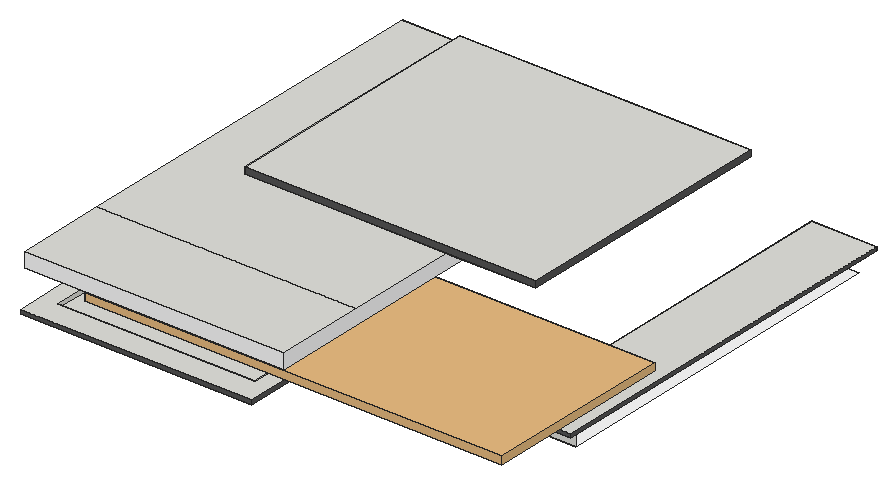
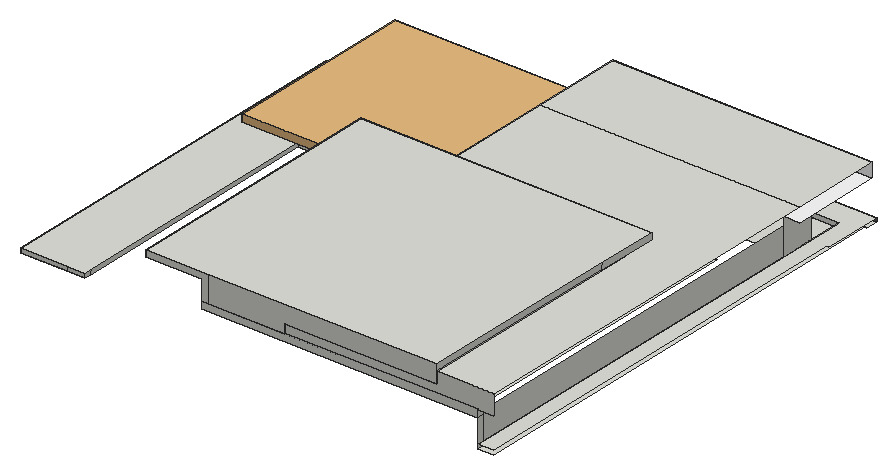
# SketchUp Ruby script. Lengths in inches.
U = 1.inch
M = Sketchup.active_model
def pt(a) = Geom::Point3d.new(a.map { |v| v * U })
def face(e, loops, mat)
  f = e.add_face(loops[0].map { |a| pt(a) })
  loops[1..].each { |l| e.add_face(l.map { |a| pt(a) }).erase! }
  f.material = f.back_material = mat if mat
  f
end
# faces: each face lists its corners as indices into pts; further lists are holes
def faces(e, pts, list, mat = nil) = list.each { |f| face(e, (f[0].is_a?(Array) ? f : [f]).map { |l| l.map { |i| pts[i] } }, mat) }
# xy, xz, yz: faces in a plane at the given z, y or x. An outline is a flat list of corners, or four numbers for a rectangle; further outlines are holes
def ring(l) = l.size == 4 ? [[l[0], l[1]], [l[2], l[1]], [l[2], l[3]], [l[0], l[3]]] : l.each_slice(2).to_a
def flat(e, list, mat, &to3) = list.each { |f| face(e, (f[0].is_a?(Array) ? f : [f]).map { |l| ring(l).map { |u, v| to3.(u, v) } }, mat) }
def xy(e, z, list, mat = nil) = flat(e, list, mat) { |x, y| [x, y, z] }
def xz(e, y, list, mat = nil) = flat(e, list, mat) { |x, z| [x, y, z] }
def yz(e, x, list, mat = nil) = flat(e, list, mat) { |y, z| [x, y, z] }
def lines(e, pts, list) = list.each { |a, b| e.add_line(pt(pts[a]), pt(pts[b])) }
# prism: a flat outline (further loops are holes) pulled along v
def prism(e, loops, v, mat = nil)
  f = face(e, loops, mat); d = Geom::Vector3d.new(v.map { |x| x * U })
  f.pushpull(f.normal.samedirection?(d) ? d.length : -d.length)
end
def box(e, o, s, mat = nil) = prism(e, [[o, [o[0] + s[0], o[1], o[2]], [o[0] + s[0], o[1] + s[1], o[2]], [o[0], o[1] + s[1], o[2]]]], [0, 0, s[2]], mat)
def at(x, y, z, deg = 0) = Geom::Transformation.translation(pt([x, y, z])) * Geom::Transformation.rotation(ORIGIN, Z_AXIS, deg.degrees)
def axes(o, x, y, z) = Geom::Transformation.new([*x, 0, *y, 0, *z, 0, *pt(o).to_a, 1])
def part(name) = M.definitions.add(name)
# library, detail: a bought-in or finely detailed component or shape, given as its bounding box
def library(name, o, s) = part(name).tap { |d| box(d.entities, o, s) }
def detail(e, o, s) = box(e.add_group.entities, o, s)
def put(e, d, t, mat = nil) = e.add_instance(d, t).tap { |i| i.material = mat if mat }
def group(e, t, mat = nil) = e.add_group.tap { |g| g.transformation = t; g.material = mat if mat }.entities
root = M.entities
M.materials.add("[Color M00]").color = [255, 255, 255]
M.materials.add("[Color M06]").color = [86, 86, 86]
c1 = library("Mesh Light\#4",[-0.5,-0.5,-0.1],[1,1,0.2])
c2 = part("Group\#24")
xy(c2.entities,0,[[203.13,95.41,201.58,95.62,200.13,96.22,198.89,97.17,197.9375,98.41,197.34,99.86,197.13,101.41,197.34,102.96,197.9375,104.41,198.89,105.65,200.13,106.61,201.58,107.21,203.13,107.41,204.6875,107.21,206.13,106.61,207.375,105.65,208.33,104.41,208.93,102.96,209.13,101.41,208.93,99.86,208.33,98.41,207.375,97.17,206.13,96.22,204.6875,95.62],[281.57,95.41,280.02,95.62,278.57,96.22,277.33,97.17,276.375,98.41,275.77,99.86,275.57,101.41,275.77,102.96,276.375,104.41,277.33,105.65,278.57,106.61,280.02,107.21,281.57,107.41,283.125,107.21,284.57,106.61,285.8125,105.65,286.77,104.41,287.37,102.96,287.57,101.41,287.37,99.86,286.77,98.41,285.8125,97.17,284.57,96.22,283.125,95.62],[350.95,95.41,349.39,95.62,347.95,96.22,346.7,97.17,345.75,98.41,345.15,99.86,344.95,101.41,345.15,102.96,345.75,104.41,346.7,105.65,347.95,106.61,349.39,107.21,350.95,107.41,352.5,107.21,353.95,106.61,355.1875,105.65,356.14,104.41,356.74,102.96,356.95,101.41,356.74,99.86,356.14,98.41,355.1875,97.17,353.95,96.22,352.5,95.62],[376,162.85,374.44,163.05,373,163.65,371.75,164.6,370.8,165.85,370.2,167.29,370,168.85,370.2,170.4,370.8,171.85,371.75,173.09,373,174.04,374.44,174.64,376,174.85,377.55,174.64,379,174.04,380.24,173.09,381.19,171.85,381.79,170.4,382,168.85,381.79,167.29,381.19,165.85,380.24,164.6,379,163.65,377.55,163.05]],"[Color M00]")
xy(c2.entities,33.4375,[[6,0,4.45,0.2,3,0.8,1.76,1.76,0.8,3,0.2,4.45,0,6,0.2,7.55,0.8,9,1.76,10.24,3,11.2,4.45,11.8,6,12,7.55,11.8,9,11.2,10.24,10.24,11.2,9,11.8,7.55,12,6,11.8,4.45,11.2,3,10.24,1.76,9,0.8,7.55,0.2],[83.125,0,81.57,0.2,80.125,0.8,78.88,1.76,77.93,3,77.33,4.45,77.125,6,77.33,7.55,77.93,9,78.88,10.24,80.125,11.2,81.57,11.8,83.125,12,84.68,11.8,86.125,11.2,87.37,10.24,88.32,9,88.92,7.55,89.125,6,88.92,4.45,88.32,3,87.37,1.76,86.125,0.8,84.68,0.2],[166.6875,0,165.13,0.2,163.6875,0.8,162.44,1.76,161.49,3,160.89,4.45,160.6875,6,160.89,7.55,161.49,9,162.44,10.24,163.6875,11.2,165.13,11.8,166.6875,12,168.24,11.8,169.6875,11.2,170.93,10.24,171.88,9,172.48,7.55,172.6875,6,172.48,4.45,171.88,3,170.93,1.76,169.6875,0.8,168.24,0.2],[166.6875,88.9375,165.13,89.14,163.6875,89.74,162.44,90.69,161.49,91.9375,160.89,93.38,160.6875,94.9375,160.89,96.49,161.49,97.9375,162.44,99.18,163.6875,100.13,165.13,100.73,166.6875,100.9375,168.24,100.73,169.6875,100.13,170.93,99.18,171.88,97.9375,172.48,96.49,172.6875,94.9375,172.48,93.38,171.88,91.9375,170.93,90.69,169.6875,89.74,168.24,89.14]],"[Color M00]")
put(c2.entities,c1,axes([191,87.42,16.72],[382.99758,0,0],[0,175.84579,0],[0,0,34.4375]))
c3 = library("Group\#23",[-0.5,-0.5,-0.1],[13,110.375,0.2])
xy(root,270.375,[[2956.13,1581.1,3168.57,1592.1],[2957.51,1592.1,2957.51,2018.36,2972.24,2018.36,2972.24,1604.38,3153.06,1604.38,3153.06,1703.22,3162.07,1703.22,3162.07,1592.1],[3162.07,1592.1,3168.57,1636.04],[2972.24,1604.38,3153.06,1604.38,3153.06,1703.22,3149.44,1703.22,3149.44,1659.57,2972.24,1659.57],[3162.07,1636.04,3168.57,1728.29],
  [3149.44,1703.22,3162.07,1773.67]])
xy(root,274.0625,[[2956.13,1581.1,3168.57,1581.1,3168.57,1673.72,3162.07,1673.72,3162.07,1703.22,3153.06,1703.22,3153.06,1604.38,2972.24,1604.38,2972.24,2018.36,2957.51,2018.36,2957.51,1636.04,2956.13,1636.04],[3162.07,1673.72,3168.57,1728.29]])
xy(root,274.0625,[[[3168.57,1673.72,3168.57,1728.29,3352.26,1728.29,3352.26,1998.71,3392.88,1998.71,3392.88,1673.72],[3203.78,1695.77,3205.34,1695.97,3206.78,1696.57,3208.03,1697.52,3208.98,1698.77,3209.58,1700.21,3209.78,1701.77,3209.58,1703.32,3208.98,1704.77,3208.03,1706.01,3206.78,1706.96,3205.34,1707.5625,3203.78,1707.77,3202.23,1707.5625,3200.78,1706.96,3199.54,1706.01,3198.59,1704.77,3197.99,1703.32,3197.78,1701.77,3197.99,1700.21,3198.59,1698.77,3199.54,1697.52,3200.78,1696.57,3202.23,1695.97],[3282.22,1695.77,3283.77,1695.97,3285.22,1696.57,3286.46,1697.52,3287.42,1698.77,3288.02,1700.21,3288.22,1701.77,3288.02,1703.32,3287.42,1704.77,3286.46,1706.01,3285.22,1706.96,3283.77,1707.5625,3282.22,1707.77,3280.67,1707.5625,3279.22,1706.96,3277.98,1706.01,3277.03,1704.77,3276.43,1703.32,3276.22,1701.77,3276.43,1700.21,3277.03,1698.77,3277.98,1697.52,3279.22,1696.57,3280.67,1695.97],[3351.6,1695.77,3353.15,1695.97,3354.6,1696.57,3355.84,1697.52,3356.79,1698.77,3357.39,1700.21,3357.6,1701.77,3357.39,1703.32,3356.79,1704.77,3355.84,1706.01,3354.6,1706.96,3353.15,1707.5625,3351.6,1707.77,3350.04,1707.5625,3348.6,1706.96,3347.35,1706.01,3346.4,1704.77,3345.8,1703.32,3345.6,1701.77,3345.8,1700.21,3346.4,1698.77,3347.35,1697.52,3348.6,1696.57,3350.04,1695.97],[3376.65,1843.64,3378.2,1843.84,3379.65,1844.44,3380.89,1845.39,3381.85,1846.64,3382.44,1848.08,3382.65,1849.64,3382.44,1851.19,3381.85,1852.64,3380.89,1853.88,3379.65,1854.83,3378.2,1855.43,3376.65,1855.64,3375.1,1855.43,3373.65,1854.83,3372.41,1853.88,3371.45,1852.64,3370.85,1851.19,3370.65,1849.64,3370.85,1848.08,3371.45,1846.64,3372.41,1845.39,3373.65,1844.44,3375.1,1843.84],[3376.65,1763.2,3378.2,1763.4,3379.65,1764,3380.89,1764.96,3381.85,1766.2,3382.44,1767.65,3382.65,1769.2,3382.44,1770.75,3381.85,1772.2,3380.89,1773.44,3379.65,1774.4,3378.2,1774.99,3376.65,1775.2,3375.1,1774.99,3373.65,1774.4,3372.41,1773.44,3371.45,1772.2,3370.85,1770.75,3370.65,1769.2,3370.85,1767.65,3371.45,1766.2,3372.41,1764.96,3373.65,1764,3375.1,1763.4],[3376.65,1941.01,3378.2,1941.22,3379.65,1941.82,3380.89,1942.77,3381.85,1944.01,3382.44,1945.46,3382.65,1947.01,3382.44,1948.56,3381.85,1950.01,3380.89,1951.25,3379.65,1952.21,3378.2,1952.81,3376.65,1953.01,3375.1,1952.81,3373.65,1952.21,3372.41,1951.25,3371.45,1950.01,3370.85,1948.56,3370.65,1947.01,3370.85,1945.46,3371.45,1944.01,3372.41,1942.77,3373.65,1941.82,3375.1,1941.22]]],"[Color M00]")
xy(root,283.9375,[[3162.07,1667.47,3392.88,1673.72],[3162.07,1673.72,3162.07,1773.67,3333.43,1773.67,3333.43,2018.36,3392.88,2018.36,3392.88,1673.72]])
xy(root,287.375,[[3162.07,1667.47,3392.88,1667.47,3392.88,2018.36,3333.43,2018.36,3333.43,1773.67,3162.07,1773.67]])
xy(root,295.8125,[[2982.55,1730.8,2982.55,2011.98,3149.44,2011.98,3149.44,1851.54,3139.92,1851.54,3139.92,1730.8],[3149.44,1851.54,3219.88,2011.98]])
xy(root,302.5625,[[2972.24,2011.98,3149.44,2018.36],[3149.44,2011.98,3219.88,2018.36]])
xy(root,307.5,[[[2957.51,1584.22,2957.51,1667.53,2972.24,1667.53,2972.24,1636.22,3149.44,1636.22,3149.44,1829.17,3195.88,1829.17,3195.88,1584.22],[3006.65,1600.35,3008.2,1600.56,3009.65,1601.16,3010.89,1602.11,3011.85,1603.35,3012.45,1604.8,3012.65,1606.35,3012.45,1607.91,3011.85,1609.35,3010.89,1610.6,3009.65,1611.55,3008.2,1612.15,3006.65,1612.35,3005.1,1612.15,3003.65,1611.55,3002.41,1610.6,3001.46,1609.35,3000.86,1607.91,3000.65,1606.35,3000.86,1604.8,3001.46,1603.35,3002.41,1602.11,3003.65,1601.16,3005.1,1600.56],[3083.78,1600.35,3085.33,1600.56,3086.78,1601.16,3088.02,1602.11,3088.97,1603.35,3089.57,1604.8,3089.78,1606.35,3089.57,1607.91,3088.97,1609.35,3088.02,1610.6,3086.78,1611.55,3085.33,1612.15,3083.78,1612.35,3082.22,1612.15,3080.78,1611.55,3079.53,1610.6,3078.58,1609.35,3077.98,1607.91,3077.78,1606.35,3077.98,1604.8,3078.58,1603.35,3079.53,1602.11,3080.78,1601.16,3082.22,1600.56],[3167.34,1689.29,3168.89,1689.5,3170.34,1690.09,3171.58,1691.05,3172.54,1692.29,3173.13,1693.74,3173.34,1695.29,3173.13,1696.84,3172.54,1698.29,3171.58,1699.53,3170.34,1700.49,3168.89,1701.09,3167.34,1701.29,3165.79,1701.09,3164.34,1700.49,3163.1,1699.53,3162.14,1698.29,3161.54,1696.84,3161.34,1695.29,3161.54,1693.74,3162.14,1692.29,3163.1,1691.05,3164.34,1690.09,3165.79,1689.5],[3167.34,1600.35,3168.89,1600.56,3170.34,1601.16,3171.58,1602.11,3172.54,1603.35,3173.13,1604.8,3173.34,1606.35,3173.13,1607.91,3172.54,1609.35,3171.58,1610.6,3170.34,1611.55,3168.89,1612.15,3167.34,1612.35,3165.79,1612.15,3164.34,1611.55,3163.1,1610.6,3162.14,1609.35,3161.54,1607.91,3161.34,1606.35,3161.54,1604.8,3162.14,1603.35,3163.1,1602.11,3164.34,1601.16,3165.79,1600.56]]],"[Color M00]")
xy(root,310.3125,[[3009.88,1829.17,3149.44,2018.36]])
xy(root,320.75,[[2957.51,1584.22,3195.88,1667.53],[2957.51,1667.53,3195.88,1667.53,3195.88,1771.54,3009.88,1771.54,3009.88,2018.36,2957.51,2018.36],[3195.88,1771.54,3195.88,1829.17,3225.88,1829.17,3225.88,2018.36,3277.44,2018.36,3277.44,1771.54]])
xy(root,326.5,[[3009.88,1771.54,3277.44,2018.36]])
xz(root,1581.1,[[2956.13,270.375,3168.57,274.0625]],"[Color M06]")
xz(root,1584.22,[[2957.51,307.5,3195.88,320.75]],"[Color M00]")
xz(root,1604.38,[[2972.24,270.375,3153.06,274.0625]])
xz(root,1667.47,[[3162.07,283.9375,3392.88,287.375]],"[Color M06]")
xz(root,1673.72,[[3162.07,274.0625,3392.88,283.9375]])
xz(root,1703.22,[[3153.06,270.375,3162.07,274.0625]])
xz(root,1771.54,[[3009.88,320.75,3277.44,326.5]],"[Color M06]")
xz(root,1773.67,[[3162.07,283.9375,3333.43,287.375]])
xz(root,1829.17,[[3149.44,307.5,3195.88,310.3125]])
xz(root,2011.98,[[2972.24,295.8125,3149.44,302.5625],[3149.44,295.8125,3219.88,302.5625]])
xz(root,2018.36,[[3333.43,283.9375,3349.13,287.375],[3349.13,283.9375,3392.88,287.375],[2972.24,295.8125,3225.88,302.5625],[2957.51,302.5625,2957.51,320.75,3009.88,320.75,3009.88,310.3125,3149.44,310.3125,3149.44,302.5625],[3149.44,302.5625,3149.44,310.3125,3009.88,310.3125,3009.88,326.5,3219.88,326.5,3219.88,302.5625],
  [3219.88,302.5625,3219.88,326.5,3277.44,326.5,3277.44,320.75,3225.88,320.75,3225.88,302.5625]])
yz(root,2972.24,[[1604.38,270.375,1636.22,274.0625],[1636.22,270.375,1659.57,274.0625],[1659.57,270.375,1667.53,274.0625],[1667.53,270.375,2011.98,274.0625],[2011.98,270.375,2018.36,274.0625],
  [1636.22,274.0625,1667.53,307.5],[1667.53,274.0625,2011.98,299.625],[2011.98,274.0625,2018.36,295.8125],[2011.98,295.8125,2018.36,302.5625]])
yz(root,3009.88,[[1801.17,310.3125,1829.17,320.75],[1829.17,310.3125,2018.36,320.75],[1771.54,320.75,1829.17,326.5],[1829.17,320.75,2018.36,326.5]])
yz(root,3149.44,[[1829.17,295.8125,2011.98,302.5625],[1829.17,302.5625,2018.36,310.3125]])
yz(root,3153.06,[[1604.38,270.375,1703.22,274.0625]])
yz(root,3162.07,[[1728.29,270.375,1728.29,274.0625,1673.72,274.0625,1673.72,283.9375,1773.67,283.9375,1773.67,270.375],[1703.22,270.375,1728.29,274.0625],[1667.47,283.9375,1773.67,287.375]])
yz(root,3168.57,[[1581.1,270.375,1728.29,274.0625]],"[Color M06]")
yz(root,3195.88,[[1584.22,307.5,1829.17,320.75]],"[Color M00]")
yz(root,3277.44,[[1771.54,320.75,2018.36,326.5]],"[Color M06]")
yz(root,3333.43,[[1773.67,283.9375,2011.98,287.375],[2011.98,283.9375,2018.36,287.375]])
yz(root,3392.88,[[1667.47,283.9375,2018.36,287.375]],"[Color M06]")
p = [[3203.78,1695.77,274.0625],[3202.23,1695.97,274.0625],[3202.23,1695.97,274.75],[3203.78,1695.77,274.75],[3205.34,1695.97,274.0625],[3205.34,1695.97,274.75],
  [3282.22,1695.77,274.0625],[3280.67,1695.97,274.0625],[3280.67,1695.97,274.75],[3282.22,1695.77,274.75],[3283.77,1695.97,274.0625],[3283.77,1695.97,274.75],
  [3351.6,1695.77,274.0625],[3350.04,1695.97,274.0625],[3350.04,1695.97,274.75],[3351.6,1695.77,274.75],[3353.15,1695.97,274.0625],[3353.15,1695.97,274.75],
  [3200.78,1696.57,274.0625],[3200.78,1696.57,274.75],[3206.78,1696.57,274.0625],[3206.78,1696.57,274.75],[3279.22,1696.57,274.0625],[3279.22,1696.57,274.75],
  [3285.22,1696.57,274.0625],[3285.22,1696.57,274.75],[3348.6,1696.57,274.0625],[3348.6,1696.57,274.75],[3354.6,1696.57,274.0625],[3354.6,1696.57,274.75],
  [3199.54,1697.52,274.0625],[3199.54,1697.52,274.75],[3208.03,1697.52,274.0625],[3208.03,1697.52,274.75],[3277.98,1697.52,274.0625],[3277.98,1697.52,274.75],
  [3286.46,1697.52,274.0625],[3286.46,1697.52,274.75],[3347.35,1697.52,274.0625],[3347.35,1697.52,274.75],[3355.84,1697.52,274.0625],[3355.84,1697.52,274.75],
  [3198.59,1698.77,274.0625],[3198.59,1698.77,274.75],[3208.98,1698.77,274.0625],[3208.98,1698.77,274.75],[3277.03,1698.77,274.0625],[3277.03,1698.77,274.75],
  [3287.42,1698.77,274.0625],[3287.42,1698.77,274.75],[3346.4,1698.77,274.0625],[3346.4,1698.77,274.75],[3356.79,1698.77,274.0625],[3356.79,1698.77,274.75],
  [3197.99,1700.21,274.0625],[3197.99,1700.21,274.75],[3209.58,1700.21,274.0625],[3209.58,1700.21,274.75],[3276.43,1700.21,274.0625],[3276.43,1700.21,274.75],
  [3288.02,1700.21,274.0625],[3288.02,1700.21,274.75],[3345.8,1700.21,274.0625],[3345.8,1700.21,274.75],[3357.39,1700.21,274.0625],[3357.39,1700.21,274.75],
  [3197.78,1701.77,274.0625],[3197.78,1701.77,274.75],[3209.78,1701.77,274.0625],[3209.78,1701.77,274.75],[3276.22,1701.77,274.0625],[3276.22,1701.77,274.75],
  [3288.22,1701.77,274.0625],[3288.22,1701.77,274.75],[3345.6,1701.77,274.0625],[3345.6,1701.77,274.75],[3357.6,1701.77,274.0625],[3357.6,1701.77,274.75],
  [3197.99,1703.32,274.0625],[3197.99,1703.32,274.75],[3209.58,1703.32,274.0625],[3209.58,1703.32,274.75],[3276.43,1703.32,274.0625],[3276.43,1703.32,274.75],
  [3288.02,1703.32,274.0625],[3288.02,1703.32,274.75],[3345.8,1703.32,274.0625],[3345.8,1703.32,274.75],[3357.39,1703.32,274.0625],[3357.39,1703.32,274.75],
  [3198.59,1704.77,274.0625],[3198.59,1704.77,274.75],[3208.98,1704.77,274.0625],[3208.98,1704.77,274.75],[3277.03,1704.77,274.0625],[3277.03,1704.77,274.75],
  [3287.42,1704.77,274.0625],[3287.42,1704.77,274.75],[3346.4,1704.77,274.0625],[3346.4,1704.77,274.75],[3356.79,1704.77,274.0625],[3356.79,1704.77,274.75],
  [3199.54,1706.01,274.0625],[3199.54,1706.01,274.75],[3208.03,1706.01,274.0625],[3208.03,1706.01,274.75],[3277.98,1706.01,274.0625],[3277.98,1706.01,274.75],
  [3286.46,1706.01,274.0625],[3286.46,1706.01,274.75],[3347.35,1706.01,274.0625],[3347.35,1706.01,274.75],[3355.84,1706.01,274.0625],[3355.84,1706.01,274.75],
  [3200.78,1706.96,274.0625],[3200.78,1706.96,274.75],[3206.78,1706.96,274.0625],[3206.78,1706.96,274.75],[3279.22,1706.96,274.0625],[3279.22,1706.96,274.75],
  [3285.22,1706.96,274.0625],[3285.22,1706.96,274.75],[3348.6,1706.96,274.0625],[3348.6,1706.96,274.75],[3354.6,1706.96,274.0625],[3354.6,1706.96,274.75],
  [3202.23,1707.5625,274.0625],[3202.23,1707.5625,274.75],[3205.34,1707.5625,274.0625],[3205.34,1707.5625,274.75],[3280.67,1707.5625,274.0625],[3280.67,1707.5625,274.75],
  [3283.77,1707.5625,274.0625],[3283.77,1707.5625,274.75],[3350.04,1707.5625,274.0625],[3350.04,1707.5625,274.75],[3353.15,1707.5625,274.0625],[3353.15,1707.5625,274.75],
  [3203.78,1707.77,274.0625],[3203.78,1707.77,274.75],[3282.22,1707.77,274.0625],[3282.22,1707.77,274.75],[3351.6,1707.77,274.0625],[3351.6,1707.77,274.75],
  [3376.65,1763.2,274.0625],[3375.1,1763.4,274.0625],[3375.1,1763.4,274.75],[3376.65,1763.2,274.75],[3378.2,1763.4,274.0625],[3378.2,1763.4,274.75],
  [3373.65,1764,274.0625],[3373.65,1764,274.75],[3379.65,1764,274.0625],[3379.65,1764,274.75],[3372.41,1764.96,274.0625],[3372.41,1764.96,274.75],
  [3380.89,1764.96,274.0625],[3380.89,1764.96,274.75],[3371.45,1766.2,274.0625],[3371.45,1766.2,274.75],[3381.85,1766.2,274.0625],[3381.85,1766.2,274.75],
  [3370.85,1767.65,274.0625],[3370.85,1767.65,274.75],[3382.44,1767.65,274.0625],[3382.44,1767.65,274.75],[3370.65,1769.2,274.0625],[3370.65,1769.2,274.75],
  [3382.65,1769.2,274.0625],[3382.65,1769.2,274.75],[3370.85,1770.75,274.0625],[3370.85,1770.75,274.75],[3382.44,1770.75,274.0625],[3382.44,1770.75,274.75],
  [3371.45,1772.2,274.0625],[3371.45,1772.2,274.75],[3381.85,1772.2,274.0625],[3381.85,1772.2,274.75],[3372.41,1773.44,274.0625],[3372.41,1773.44,274.75],
  [3380.89,1773.44,274.0625],[3380.89,1773.44,274.75],[3373.65,1774.4,274.0625],[3373.65,1774.4,274.75],[3379.65,1774.4,274.0625],[3379.65,1774.4,274.75],
  [3375.1,1774.99,274.0625],[3375.1,1774.99,274.75],[3378.2,1774.99,274.0625],[3378.2,1774.99,274.75],[3376.65,1775.2,274.0625],[3376.65,1775.2,274.75],
  [3376.65,1843.64,274.0625],[3375.1,1843.84,274.0625],[3375.1,1843.84,274.75],[3376.65,1843.64,274.75],[3378.2,1843.84,274.0625],[3378.2,1843.84,274.75],
  [3373.65,1844.44,274.0625],[3373.65,1844.44,274.75],[3379.65,1844.44,274.0625],[3379.65,1844.44,274.75],[3372.41,1845.39,274.0625],[3372.41,1845.39,274.75],
  [3380.89,1845.39,274.0625],[3380.89,1845.39,274.75],[3371.45,1846.64,274.0625],[3371.45,1846.64,274.75],[3381.85,1846.64,274.0625],[3381.85,1846.64,274.75],
  [3370.85,1848.08,274.0625],[3370.85,1848.08,274.75],[3382.44,1848.08,274.0625],[3382.44,1848.08,274.75],[3370.65,1849.64,274.0625],[3370.65,1849.64,274.75],
  [3382.65,1849.64,274.0625],[3382.65,1849.64,274.75],[3370.85,1851.19,274.0625],[3370.85,1851.19,274.75],[3382.44,1851.19,274.0625],[3382.44,1851.19,274.75],
  [3371.45,1852.64,274.0625],[3371.45,1852.64,274.75],[3381.85,1852.64,274.0625],[3381.85,1852.64,274.75],[3372.41,1853.88,274.0625],[3372.41,1853.88,274.75],
  [3380.89,1853.88,274.0625],[3380.89,1853.88,274.75],[3373.65,1854.83,274.0625],[3373.65,1854.83,274.75],[3379.65,1854.83,274.0625],[3379.65,1854.83,274.75],
  [3375.1,1855.43,274.0625],[3375.1,1855.43,274.75],[3378.2,1855.43,274.0625],[3378.2,1855.43,274.75],[3376.65,1855.64,274.0625],[3376.65,1855.64,274.75],
  [3376.65,1941.01,274.0625],[3375.1,1941.22,274.0625],[3375.1,1941.22,274.75],[3376.65,1941.01,274.75],[3378.2,1941.22,274.0625],[3378.2,1941.22,274.75],
  [3373.65,1941.82,274.0625],[3373.65,1941.82,274.75],[3379.65,1941.82,274.0625],[3379.65,1941.82,274.75],[3372.41,1942.77,274.0625],[3372.41,1942.77,274.75],
  [3380.89,1942.77,274.0625],[3380.89,1942.77,274.75],[3371.45,1944.01,274.0625],[3371.45,1944.01,274.75],[3381.85,1944.01,274.0625],[3381.85,1944.01,274.75],
  [3370.85,1945.46,274.0625],[3370.85,1945.46,274.75],[3382.44,1945.46,274.0625],[3382.44,1945.46,274.75],[3370.65,1947.01,274.0625],[3370.65,1947.01,274.75],
  [3382.65,1947.01,274.0625],[3382.65,1947.01,274.75],[3370.85,1948.56,274.0625],[3370.85,1948.56,274.75],[3382.44,1948.56,274.0625],[3382.44,1948.56,274.75],
  [3371.45,1950.01,274.0625],[3371.45,1950.01,274.75],[3381.85,1950.01,274.0625],[3381.85,1950.01,274.75],[3372.41,1951.25,274.0625],[3372.41,1951.25,274.75],
  [3380.89,1951.25,274.0625],[3380.89,1951.25,274.75],[3373.65,1952.21,274.0625],[3373.65,1952.21,274.75],[3379.65,1952.21,274.0625],[3379.65,1952.21,274.75],
  [3375.1,1952.81,274.0625],[3375.1,1952.81,274.75],[3378.2,1952.81,274.0625],[3378.2,1952.81,274.75],[3376.65,1953.01,274.0625],[3376.65,1953.01,274.75],
  [3006.65,1600.35,307.5],[3005.1,1600.56,307.5],[3005.1,1600.56,308.1875],[3006.65,1600.35,308.1875],[3008.2,1600.56,307.5],[3008.2,1600.56,308.1875],
  [3083.78,1600.35,307.5],[3082.22,1600.56,307.5],[3082.22,1600.56,308.1875],[3083.78,1600.35,308.1875],[3085.33,1600.56,307.5],[3085.33,1600.56,308.1875],
  [3167.34,1600.35,307.5],[3165.79,1600.56,307.5],[3165.79,1600.56,308.1875],[3167.34,1600.35,308.1875],[3168.89,1600.56,307.5],[3168.89,1600.56,308.1875],
  [3003.65,1601.16,307.5],[3003.65,1601.16,308.1875],[3009.65,1601.16,307.5],[3009.65,1601.16,308.1875],[3080.78,1601.16,307.5],[3080.78,1601.16,308.1875],
  [3086.78,1601.16,307.5],[3086.78,1601.16,308.1875],[3164.34,1601.16,307.5],[3164.34,1601.16,308.1875],[3170.34,1601.16,307.5],[3170.34,1601.16,308.1875],
  [3002.41,1602.11,307.5],[3002.41,1602.11,308.1875],[3010.89,1602.11,307.5],[3010.89,1602.11,308.1875],[3079.53,1602.11,307.5],[3079.53,1602.11,308.1875],
  [3088.02,1602.11,307.5],[3088.02,1602.11,308.1875],[3163.1,1602.11,307.5],[3163.1,1602.11,308.1875],[3171.58,1602.11,307.5],[3171.58,1602.11,308.1875],
  [3001.46,1603.35,307.5],[3001.46,1603.35,308.1875],[3011.85,1603.35,307.5],[3011.85,1603.35,308.1875],[3078.58,1603.35,307.5],[3078.58,1603.35,308.1875],
  [3088.97,1603.35,307.5],[3088.97,1603.35,308.1875],[3162.14,1603.35,307.5],[3162.14,1603.35,308.1875],[3172.54,1603.35,307.5],[3172.54,1603.35,308.1875],
  [3000.86,1604.8,307.5],[3000.86,1604.8,308.1875],[3012.45,1604.8,307.5],[3012.45,1604.8,308.1875],[3077.98,1604.8,307.5],[3077.98,1604.8,308.1875],
  [3089.57,1604.8,307.5],[3089.57,1604.8,308.1875],[3161.54,1604.8,307.5],[3161.54,1604.8,308.1875],[3173.13,1604.8,307.5],[3173.13,1604.8,308.1875],
  [3000.65,1606.35,307.5],[3000.65,1606.35,308.1875],[3012.65,1606.35,307.5],[3012.65,1606.35,308.1875],[3077.78,1606.35,307.5],[3077.78,1606.35,308.1875],
  [3089.78,1606.35,307.5],[3089.78,1606.35,308.1875],[3161.34,1606.35,307.5],[3161.34,1606.35,308.1875],[3173.34,1606.35,307.5],[3173.34,1606.35,308.1875],
  [3000.86,1607.91,307.5],[3000.86,1607.91,308.1875],[3012.45,1607.91,307.5],[3012.45,1607.91,308.1875],[3077.98,1607.91,307.5],[3077.98,1607.91,308.1875],
  [3089.57,1607.91,307.5],[3089.57,1607.91,308.1875],[3161.54,1607.91,307.5],[3161.54,1607.91,308.1875],[3173.13,1607.91,307.5],[3173.13,1607.91,308.1875],
  [3001.46,1609.35,307.5],[3001.46,1609.35,308.1875],[3011.85,1609.35,307.5],[3011.85,1609.35,308.1875],[3078.58,1609.35,307.5],[3078.58,1609.35,308.1875],
  [3088.97,1609.35,307.5],[3088.97,1609.35,308.1875],[3162.14,1609.35,307.5],[3162.14,1609.35,308.1875],[3172.54,1609.35,307.5],[3172.54,1609.35,308.1875],
  [3002.41,1610.6,307.5],[3002.41,1610.6,308.1875],[3010.89,1610.6,307.5],[3010.89,1610.6,308.1875],[3079.53,1610.6,307.5],[3079.53,1610.6,308.1875],
  [3088.02,1610.6,307.5],[3088.02,1610.6,308.1875],[3163.1,1610.6,307.5],[3163.1,1610.6,308.1875],[3171.58,1610.6,307.5],[3171.58,1610.6,308.1875],
  [3003.65,1611.55,307.5],[3003.65,1611.55,308.1875],[3009.65,1611.55,307.5],[3009.65,1611.55,308.1875],[3080.78,1611.55,307.5],[3080.78,1611.55,308.1875],
  [3086.78,1611.55,307.5],[3086.78,1611.55,308.1875],[3164.34,1611.55,307.5],[3164.34,1611.55,308.1875],[3170.34,1611.55,307.5],[3170.34,1611.55,308.1875],
  [3005.1,1612.15,307.5],[3005.1,1612.15,308.1875],[3008.2,1612.15,307.5],[3008.2,1612.15,308.1875],[3082.22,1612.15,307.5],[3082.22,1612.15,308.1875],
  [3085.33,1612.15,307.5],[3085.33,1612.15,308.1875],[3165.79,1612.15,307.5],[3165.79,1612.15,308.1875],[3168.89,1612.15,307.5],[3168.89,1612.15,308.1875],
  [3006.65,1612.35,307.5],[3006.65,1612.35,308.1875],[3083.78,1612.35,307.5],[3083.78,1612.35,308.1875],[3167.34,1612.35,307.5],[3167.34,1612.35,308.1875],
  [3167.34,1689.29,307.5],[3165.79,1689.5,307.5],[3165.79,1689.5,308.1875],[3167.34,1689.29,308.1875],[3168.89,1689.5,307.5],[3168.89,1689.5,308.1875],
  [3164.34,1690.09,307.5],[3164.34,1690.09,308.1875],[3170.34,1690.09,307.5],[3170.34,1690.09,308.1875],[3163.1,1691.05,307.5],[3163.1,1691.05,308.1875],
  [3171.58,1691.05,307.5],[3171.58,1691.05,308.1875],[3162.14,1692.29,307.5],[3162.14,1692.29,308.1875],[3172.54,1692.29,307.5],[3172.54,1692.29,308.1875],
  [3161.54,1693.74,307.5],[3161.54,1693.74,308.1875],[3173.13,1693.74,307.5],[3173.13,1693.74,308.1875],[3161.34,1695.29,307.5],[3161.34,1695.29,308.1875],
  [3173.34,1695.29,307.5],[3173.34,1695.29,308.1875],[3161.54,1696.84,307.5],[3161.54,1696.84,308.1875],[3173.13,1696.84,307.5],[3173.13,1696.84,308.1875],
  [3162.14,1698.29,307.5],[3162.14,1698.29,308.1875],[3172.54,1698.29,307.5],[3172.54,1698.29,308.1875],[3163.1,1699.53,307.5],[3163.1,1699.53,308.1875],
  [3171.58,1699.53,307.5],[3171.58,1699.53,308.1875],[3164.34,1700.49,307.5],[3164.34,1700.49,308.1875],[3170.34,1700.49,307.5],[3170.34,1700.49,308.1875],
  [3165.79,1701.09,307.5],[3165.79,1701.09,308.1875],[3168.89,1701.09,307.5],[3168.89,1701.09,308.1875],[3167.34,1701.29,307.5],[3167.34,1701.29,308.1875],
  [3009.88,1801.17,310.3125],[3179.51,1801.17,310.3125],[3219.88,2011.98,302.5625],[3219.88,1829.17,302.5625],[3219.88,1851.54,295.8125],[3225.88,1851.54,295.8125],
  [3149.44,1773.67,270.375],[3149.44,1773.67,282.1875],[3352.26,1998.71,274.0625],[3352.26,1998.71,282.1875],[3219.88,1829.17,295.8125],[2982.55,1730.8,295.8125],
  [2972.24,1730.8,295.8125]]
faces(root,p,[[0,1,2,3],[4,0,3,5],[6,7,8,9],[10,6,9,11],[12,13,14,15],[16,12,15,17],[1,18,19,2],[20,4,5,21],
  [7,22,23,8],[24,10,11,25],[13,26,27,14],[28,16,17,29],[18,30,31,19],[32,20,21,33],[22,34,35,23],[36,24,25,37],
  [26,38,39,27],[40,28,29,41],[30,42,43,31],[44,32,33,45],[34,46,47,35],[48,36,37,49],[38,50,51,39],[52,40,41,53],
  [42,54,55,43],[56,44,45,57],[46,58,59,47],[60,48,49,61],[50,62,63,51],[64,52,53,65],[54,66,67,55],[68,56,57,69],
  [58,70,71,59],[72,60,61,73],[62,74,75,63],[76,64,65,77],[66,78,79,67],[80,68,69,81],[70,82,83,71],[84,72,73,85],
  [74,86,87,75],[88,76,77,89],[78,90,91,79],[92,80,81,93],[82,94,95,83],[96,84,85,97],[86,98,99,87],[100,88,89,101],
  [90,102,103,91],[104,92,93,105],[94,106,107,95],[108,96,97,109],[98,110,111,99],[112,100,101,113],[102,114,115,103],[116,104,105,117],
  [106,118,119,107],[120,108,109,121],[110,122,123,111],[124,112,113,125],[114,126,127,115],[128,116,117,129],[118,130,131,119],[132,120,121,133],
  [122,134,135,123],[136,124,125,137],[126,138,139,127],[138,128,129,139],[130,140,141,131],[140,132,133,141],[134,142,143,135],[142,136,137,143],
  [144,145,146,147],[148,144,147,149],[145,150,151,146],[152,148,149,153],[150,154,155,151],[156,152,153,157],[154,158,159,155],[160,156,157,161],
  [158,162,163,159],[164,160,161,165],[162,166,167,163],[168,164,165,169],[166,170,171,167],[172,168,169,173],[170,174,175,171],[176,172,173,177],
  [174,178,179,175],[180,176,177,181],[178,182,183,179],[184,180,181,185],[182,186,187,183],[188,184,185,189],[186,190,191,187],[190,188,189,191],
  [192,193,194,195],[196,192,195,197],[193,198,199,194],[200,196,197,201],[198,202,203,199],[204,200,201,205],[202,206,207,203],[208,204,205,209],
  [206,210,211,207],[212,208,209,213],[210,214,215,211],[216,212,213,217],[214,218,219,215],[220,216,217,221],[218,222,223,219],[224,220,221,225],
  [222,226,227,223],[228,224,225,229],[226,230,231,227],[232,228,229,233],[230,234,235,231],[236,232,233,237],[234,238,239,235],[238,236,237,239],
  [240,241,242,243],[244,240,243,245],[241,246,247,242],[248,244,245,249],[246,250,251,247],[252,248,249,253],[250,254,255,251],[256,252,253,257],
  [254,258,259,255],[260,256,257,261],[258,262,263,259],[264,260,261,265],[262,266,267,263],[268,264,265,269],[266,270,271,267],[272,268,269,273],
  [270,274,275,271],[276,272,273,277],[274,278,279,275],[280,276,277,281],[278,282,283,279],[284,280,281,285],[282,286,287,283],[286,284,285,287],
  [288,289,290,291],[292,288,291,293],[294,295,296,297],[298,294,297,299],[300,301,302,303],[304,300,303,305],[289,306,307,290],[308,292,293,309],
  [295,310,311,296],[312,298,299,313],[301,314,315,302],[316,304,305,317],[306,318,319,307],[320,308,309,321],[310,322,323,311],[324,312,313,325],
  [314,326,327,315],[328,316,317,329],[318,330,331,319],[332,320,321,333],[322,334,335,323],[336,324,325,337],[326,338,339,327],[340,328,329,341],
  [330,342,343,331],[344,332,333,345],[334,346,347,335],[348,336,337,349],[338,350,351,339],[352,340,341,353],[342,354,355,343],[356,344,345,357],
  [346,358,359,347],[360,348,349,361],[350,362,363,351],[364,352,353,365],[354,366,367,355],[368,356,357,369],[358,370,371,359],[372,360,361,373],
  [362,374,375,363],[376,364,365,377],[366,378,379,367],[380,368,369,381],[370,382,383,371],[384,372,373,385],[374,386,387,375],[388,376,377,389],
  [378,390,391,379],[392,380,381,393],[382,394,395,383],[396,384,385,397],[386,398,399,387],[400,388,389,401],[390,402,403,391],[404,392,393,405],
  [394,406,407,395],[408,396,397,409],[398,410,411,399],[412,400,401,413],[402,414,415,403],[416,404,405,417],[406,418,419,407],[420,408,409,421],
  [410,422,423,411],[424,412,413,425],[414,426,427,415],[426,416,417,427],[418,428,429,419],[428,420,421,429],[422,430,431,423],[430,424,425,431],
  [432,433,434,435],[436,432,435,437],[433,438,439,434],[440,436,437,441],[438,442,443,439],[444,440,441,445],[442,446,447,443],[448,444,445,449],
  [446,450,451,447],[452,448,449,453],[450,454,455,451],[456,452,453,457],[454,458,459,455],[460,456,457,461],[458,462,463,459],[464,460,461,465],
  [462,466,467,463],[468,464,465,469],[466,470,471,467],[472,468,469,473],[470,474,475,471],[476,472,473,477],[474,478,479,475],[478,476,477,479]],"[Color M00]")
lines(root,p,[[480,481],[482,483],[484,485],[486,487],[488,489],[484,490],[491,492]])
put(root,c2,at(3000.65,1600.35,274.75))
put(root,c3,at(3370.65,1843.64,274.75))
